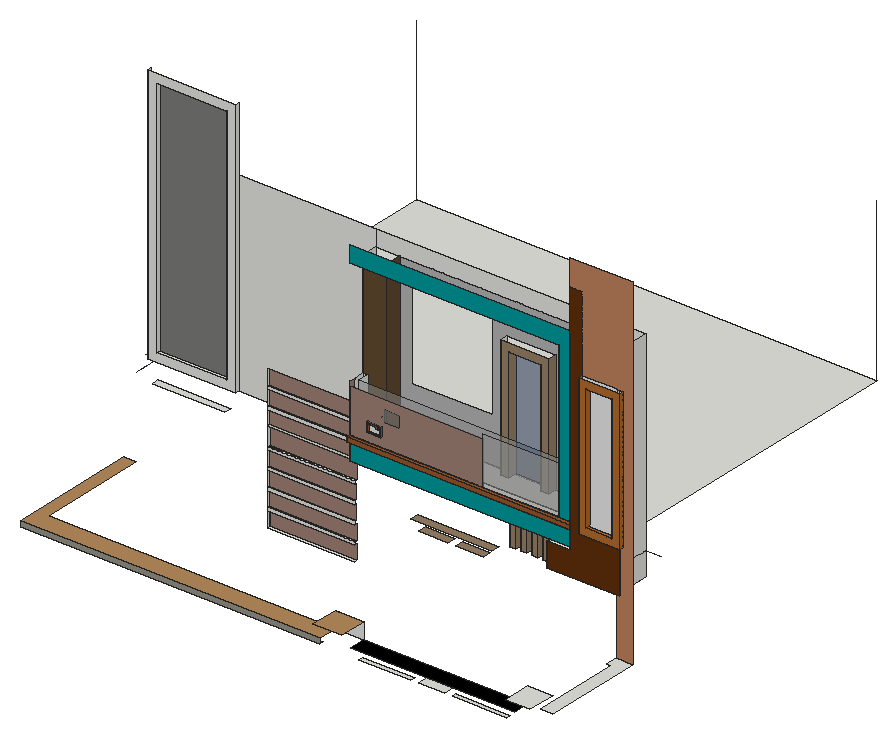
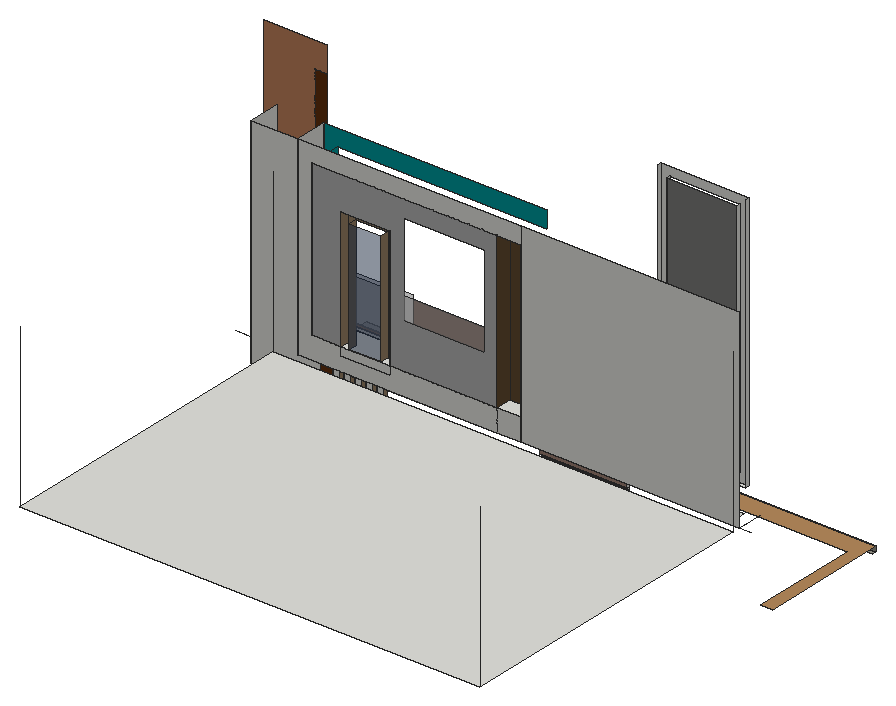
# SketchUp Ruby script. Lengths in inches.
U = 1.inch
M = Sketchup.active_model
def pt(a) = Geom::Point3d.new(a.map { |v| v * U })
def face(e, loops, mat)
  f = e.add_face(loops[0].map { |a| pt(a) })
  loops[1..].each { |l| e.add_face(l.map { |a| pt(a) }).erase! }
  f.material = f.back_material = mat if mat
  f
end
# faces: each face lists its corners as indices into pts; further lists are holes
def faces(e, pts, list, mat = nil) = list.each { |f| face(e, (f[0].is_a?(Array) ? f : [f]).map { |l| l.map { |i| pts[i] } }, mat) }
# xy, xz, yz: faces in a plane at the given z, y or x. An outline is a flat list of corners, or four numbers for a rectangle; further outlines are holes
def ring(l) = l.size == 4 ? [[l[0], l[1]], [l[2], l[1]], [l[2], l[3]], [l[0], l[3]]] : l.each_slice(2).to_a
def flat(e, list, mat, &to3) = list.each { |f| face(e, (f[0].is_a?(Array) ? f : [f]).map { |l| ring(l).map { |u, v| to3.(u, v) } }, mat) }
def xy(e, z, list, mat = nil) = flat(e, list, mat) { |x, y| [x, y, z] }
def xz(e, y, list, mat = nil) = flat(e, list, mat) { |x, z| [x, y, z] }
def yz(e, x, list, mat = nil) = flat(e, list, mat) { |y, z| [x, y, z] }
def lines(e, pts, list) = list.each { |a, b| e.add_line(pt(pts[a]), pt(pts[b])) }
# prism: a flat outline (further loops are holes) pulled along v
def prism(e, loops, v, mat = nil)
  f = face(e, loops, mat); d = Geom::Vector3d.new(v.map { |x| x * U })
  f.pushpull(f.normal.samedirection?(d) ? d.length : -d.length)
end
def box(e, o, s, mat = nil) = prism(e, [[o, [o[0] + s[0], o[1], o[2]], [o[0] + s[0], o[1] + s[1], o[2]], [o[0], o[1] + s[1], o[2]]]], [0, 0, s[2]], mat)
def at(x, y, z, deg = 0) = Geom::Transformation.translation(pt([x, y, z])) * Geom::Transformation.rotation(ORIGIN, Z_AXIS, deg.degrees)
def axes(o, x, y, z) = Geom::Transformation.new([*x, 0, *y, 0, *z, 0, *pt(o).to_a, 1])
def part(name) = M.definitions.add(name)
# library, detail: a bought-in or finely detailed component or shape, given as its bounding box
def library(name, o, s) = part(name).tap { |d| box(d.entities, o, s) }
def detail(e, o, s) = box(e.add_group.entities, o, s)
def put(e, d, t, mat = nil) = e.add_instance(d, t).tap { |i| i.material = mat if mat }
def group(e, t, mat = nil) = e.add_group.tap { |g| g.transformation = t; g.material = mat if mat }.entities
root = M.entities
M.materials.add("Niraj_Hair_Gray").color = [178, 178, 178]
M.materials.add("Niraj_Shoe_Sole").color = [96, 73, 48]
M.materials.add("Niraj_Shoe_Stitching").color = [181, 137, 92]
M.materials.add("Niraj_Skin").color = [158, 128, 115]
M.materials.add("[0035_Tan]").color = [150, 128, 100]
M.materials.add("[0043_SaddleBrown]").color = [96, 48, 13]
M.materials.add("[0083_DarkTurquoise]").color = [0, 153, 155]
M.materials.add("[0137_Black]").color = [0, 0, 0]
M.materials.add("[Basketweave]").color = [230, 230, 230]
M.materials.add("[Encaustic Tile Circular 01]").color = [123, 123, 122]
M.materials.add("[Formica Graystone]").color = [149, 146, 135]
M.materials.add("[Marble Carrara Gold Floor Tile]").color = [225, 223, 217]
M.materials.add("[Translucent Glass Blue]").color = [40, 60, 96]
M.materials["[Translucent Glass Blue]"].alpha = 0.5
M.materials.add("[Translucent Glass Gray]").color = [165, 165, 165]
M.materials["[Translucent Glass Gray]"].alpha = 0.5
M.materials.add("[Wood Bamboo]").color = [177, 105, 43]
M.materials.add("[Wood Cherry Original]").color = [152, 86, 42]
M.materials.add("[Wood Veneer 02]").color = [190, 128, 91]
xy(root,50.7,[[106.63,122.375,171.63,124.5]])
xy(root,54,[[249.65,28.875,288.24,31.875],[294.24,28.875,313.08,40.875],[319.08,28.875,359.58,31.875]])
xy(root,56.2,[[0,25.875,222.65,28.875]],"[Formica Graystone]")
xy(root,60,[[375,40.875,384,40.875,384,115,372,115,372,106,375,106]])
xy(root,60,[[0,25.875,222.65,25.875,222.65,40.875,9,40.875,9,122.375,0,122.375]],"Niraj_Shoe_Stitching")
xy(root,60,[[243.65,28.875,365.58,40.875]],"[0137_Black]")
xy(root,61.77,[[106.63,122.375,171.63,124.5]])
xy(root,64.2,[[106.63,122.375,171.63,123.875]])
xy(root,72,[[365.58,19.875,384,40.875]])
xy(root,72,[[222.65,19.875,243.65,40.875]],"Niraj_Shoe_Stitching")
xy(root,75.27,[[106.63,122.375,171.63,123.875]])
xy(root,77.7,[[106.63,122.375,171.63,123.5625]])
xy(root,78,[[208.6,136,229.96,142],[235.96,136,256.6,142]],"[0035_Tan]")
xy(root,84,[[202.6,136,262.6,142]],"[0035_Tan]")
xy(root,88.77,[[106.63,122.375,171.63,123.5625]])
xy(root,89.375,[[273.47,139,278.35,142],[281.66,139,286.54,142],[289.85,139,294.72,142],[298.04,139,302.91,142],[306.22,139,311.1,142]],"[0035_Tan]")
xy(root,91.2,[[106.63,122.375,171.63,123.5]])
xy(root,102.25,[[372,115,374.5,118]])
xy(root,102.25,[[320.38,115,372,142]],"[0043_SaddleBrown]")
xy(root,102.27,[[106.63,122.375,171.63,123.5]])
xy(root,104.7,[[106.63,122.375,171.63,123.9375],[106.63,123.9375,171.63,124.1875]])
xy(root,116.62,[[21.24,122.375,75.18,127.1875]])
xy(root,118.2,[[106.63,122.375,171.63,123.6875],[106.63,123.6875,171.63,124.1875]])
xy(root,120,[[320.38,115,337.38,118],[171.63,118,189.04,130],[320.38,118,337.38,142],[171.63,130,189.04,142],[273.47,139,278.35,142],
  [281.66,139,286.54,142],[289.85,139,294.72,142],[298.04,139,302.91,142],[306.22,139,311.1,142],[9,148,351,382.875]])
xy(root,120,[[189.04,118,189.04,142,273.47,142,273.47,139,278.35,139,278.35,142,281.66,142,281.66,139,286.54,139,286.54,142,289.85,142,289.85,139,294.72,139,294.72,142,298.04,142,298.04,139,302.91,139,302.91,142,306.22,142,306.22,139,311.1,139,311.1,142,320.38,142,320.38,118]],"[0083_DarkTurquoise]")
xy(root,129.27,[[106.63,122.375,171.63,123.6875]])
xy(root,131.7,[[106.63,122.375,171.63,123.9375]])
xy(root,133.71,[[171.63,115,337.38,118]],"[Wood Cherry Original]")
xy(root,134.02,[[20.16,119.375,85.33,122.375]])
xy(root,135.45,[[346.46,115,374.5,118],[374.5,115,376.65,118]])
xy(root,135.45,[[346.46,112,376.65,115]],"[Wood Bamboo]")
xy(root,136.875,[[171.63,118,171.63,130,175.07,130,175.07,122.125,326.57,122.125,326.57,118],[171.63,130,189.04,142],[269.26,136,275.26,142],[299.26,136,305.26,142]])
xy(root,136.875,[[175.07,122.125,326.57,122.125,326.57,142,305.26,142,305.26,136,299.26,136,299.26,142,275.26,142,275.26,136,269.26,136,269.26,142,189.04,142,189.04,130,175.07,130]],"[Marble Carrara Gold Floor Tile]")
xy(root,136.875,[[171.63,115,337.38,118]],"[Wood Cherry Original]")
xy(root,140.38,[[26.53,119.375,78.96,122.375]])
xy(root,140.875,[[351.89,112,371.22,118]],"[Wood Bamboo]")
xy(root,142.77,[[106.63,122.375,171.63,123.9375]])
xy(root,144.11,[[184.65,117,195.37,118]],"[Wood Cherry Original]")
xy(root,144.68,[[185.22,117,194.8,118]],"[Wood Cherry Original]")
xy(root,145.2,[[106.63,122.375,171.63,123.3125]])
xz(root,25.875,[[0,56.2,222.65,60]],"[Formica Graystone]")
xz(root,40.875,[[222.65,60,243.65,72]])
xz(root,112,[[[346.46,135.45,376.65,239.26],[351.89,140.875,371.22,233.83]]],"[Wood Bamboo]")
xz(root,115,[[372,135.45,374.5,239.26],[374.5,135.45,376.65,239.26]])
xz(root,115,[[320.38,102.25,374.5,102.25,374.5,135.45,346.46,135.45,346.46,295.34,337.38,295.34,337.38,120,320.38,120]],"[0043_SaddleBrown]")
xz(root,115,[[346.46,135.45,372,239.26]],"[Basketweave]")
xz(root,115,[[171.63,133.71,337.38,136.875]],"[Wood Cherry Original]")
xz(root,115,[[372,60,384,60,384,314.9,337.38,314.9,337.38,295.34,346.46,295.34,346.46,239.26,376.65,239.26,376.65,135.45,374.5,135.45,374.5,102.25,372,102.25]],"[Wood Veneer 02]")
xz(root,117,[[[184.65,144.11,195.37,150.73],[185.22,144.68,185.22,150.16,191.85,150.16,191.85,148.76,194.8,148.76,194.8,144.68],[192.49,149.21,194.8,150.16]]],"[Wood Cherry Original]")
xz(root,118,[[371.25,102.25,372,135.45],[372,102.25,374.5,135.45],[171.63,133.71,337.38,136.875],[346.46,135.45,371.25,239.26],[371.25,135.45,372,239.26],
  [372,135.45,374.5,239.26],[374.5,135.45,376.65,239.26],[351.89,140.875,371.22,233.83],[185.22,144.68,194.8,144.68,194.8,148.76,191.85,148.76,191.85,150.16,185.22,150.16]])
xz(root,118,[[[171.63,136.875,270.57,169.5625],[184.65,144.11,184.65,150.73,191.85,150.73,191.85,157.63,196.34,157.63,196.34,163.04,208.53,163.04,208.53,153.79,196.34,153.79,196.34,157.01,196.95,157.02,192.49,157.02,192.49,150.73,195.37,150.73,195.37,144.11]]],"Niraj_Skin")
xz(root,118,[[171.63,120,337.38,133.71],[326.57,136.875,337.38,136.875,337.38,264,171.63,264,171.63,251.8,326.57,251.8]],"[0083_DarkTurquoise]")
xz(root,118,[[270.57,136.875,326.57,172.875]],"[Translucent Glass Gray]")
xz(root,119.375,[[[20.16,134.02,85.33,326.3125],[26.53,140.38,78.96,319.95]]])
xz(root,122.125,[[175.07,136.875,326.57,172.875]],"[Translucent Glass Gray]")
xz(root,122.375,[[106.63,61.77,171.63,64.2],[106.63,75.27,171.63,77.7],[106.63,88.77,171.63,91.2],[106.63,102.27,171.63,104.7],[106.63,118.2,171.63,120],
  [106.63,129.27,171.63,131.7],[106.63,142.77,171.63,145.2]])
xz(root,122.375,[[26.53,140.38,78.96,319.95]],"[Encaustic Tile Circular 01]")
xz(root,123.3125,[[106.63,145.2,171.63,156.27]],"Niraj_Skin")
xz(root,123.5,[[106.63,91.2,171.63,102.27]],"Niraj_Skin")
xz(root,123.5625,[[106.63,77.7,171.63,88.77]],"Niraj_Skin")
xz(root,123.6875,[[106.63,118.2,171.63,129.27]],"Niraj_Skin")
xz(root,123.875,[[106.63,64.2,171.63,75.27]],"Niraj_Skin")
xz(root,123.9375,[[106.63,131.7,171.63,142.77]],"Niraj_Skin")
xz(root,124.1875,[[106.63,104.7,171.63,118.2]],"Niraj_Skin")
xz(root,124.5,[[106.63,50.7,171.63,61.77]],"Niraj_Skin")
xz(root,130,[[171.63,136.875,175.07,172.875]])
xz(root,130,[[175.07,136.875,189.04,136.875,189.04,251.8,171.63,251.8,171.63,172.875,175.07,172.875]],"Niraj_Shoe_Sole")
xz(root,136,[[269.26,136.875,275.26,136.875,275.26,220.875,299.26,220.875,299.26,136.875,305.26,136.875,305.26,226.875,269.26,226.875]],"[0035_Tan]")
xz(root,139,[[273.47,89.375,278.35,120],[281.66,89.375,286.54,120],[289.85,89.375,294.72,120],[298.04,89.375,302.91,120],[306.22,89.375,311.1,120]],"[0035_Tan]")
xz(root,142,[[273.47,89.375,278.35,120],[281.66,89.375,286.54,120],[289.85,89.375,294.72,120],[298.04,89.375,302.91,120],[306.22,89.375,311.1,120],
  [320.38,102.25,320.38,120,337.38,120,337.38,264,372,264,372,102.25],[9,120,171.63,264],[171.63,120,189.04,136.875],[189.04,120,337.38,120,337.38,264,171.63,264,171.63,251.8,326.57,251.8,326.57,136.875,305.26,136.875,305.26,130.875,269.26,130.875,269.26,136.875,189.04,136.875],[269.26,130.875,305.26,136.875]])
xz(root,142,[[[189.04,136.875,269.26,136.875,269.26,226.875,305.26,226.875,305.26,136.875,326.57,136.875,326.57,251.8,189.04,251.8],[198.26,170.25,258.45,239]]],"Niraj_Hair_Gray")
xz(root,142,[[275.26,136.875,299.26,220.875]],"[Translucent Glass Blue]")
yz(root,20.16,[[119.375,134.02,122.375,326.3125]])
yz(root,26.53,[[119.375,140.38,122.375,319.95]])
yz(root,78.96,[[119.375,140.38,122.375,319.95]])
yz(root,85.33,[[119.375,134.02,122.375,326.3125]])
yz(root,106.63,[[122.375,50.7,123.9375,61.77],[123.9375,50.7,124.5,61.77],[122.375,64.2,123.875,75.27],[123.875,64.2,124.5625,75.27],[122.375,77.7,123.5625,88.77],
  [123.5625,77.7,124.125,88.77],[122.375,91.2,123.5,102.27],[123.5,91.2,124.125,102.27],[122.375,104.7,124.1875,118.2],[122.375,118.2,123.6875,129.27],
  [122.375,131.7,123.9375,142.77],[122.375,145.2,123.3125,156.27]])
yz(root,171.63,[[122.375,118.2,123.6875,120],[123.6875,120,142,120,142,136.875,123.9375,136.875,123.9375,131.7,122.375,131.7,122.375,129.27,123.6875,129.27],[123.9375,136.875,123.9375,142.77,122.375,142.77,122.375,145.2,123.3125,145.2,123.3125,156.27,122.375,156.27,122.375,172.875,130,172.875,130,136.875],[130,136.875,142,251.8]])
yz(root,171.63,[[118,136.875,118,172.875,122.375,172.875,122.375,156.27,123.3125,156.27,123.3125,145.2,122.375,145.2,122.375,142.77,123.9375,142.77,123.9375,136.875]],"Niraj_Skin")
yz(root,171.63,[[118,120,118,136.875,123.9375,136.875,123.9375,131.7,122.375,131.7,122.375,129.27,123.6875,129.27,123.6875,120]],"[0083_DarkTurquoise]")
yz(root,171.63,[[115,133.71,118,136.875]],"[Wood Cherry Original]")
yz(root,175.07,[[122.125,136.875,130,172.875]])
yz(root,184.65,[[117,144.11,118,150.73]],"[Wood Cherry Original]")
yz(root,185.22,[[117,144.68,118,150.16]],"[Wood Cherry Original]")
yz(root,189.04,[[130,136.875,142,251.8]],"Niraj_Shoe_Sole")
yz(root,194.8,[[117,144.68,118,148.76]],"[Wood Cherry Original]")
yz(root,195.37,[[117,144.11,118,150.73]],"[Wood Cherry Original]")
yz(root,269.26,[[136,136.875,142,226.875]])
yz(root,273.47,[[139,89.375,142,120]],"[0035_Tan]")
yz(root,275.26,[[136,136.875,142,220.875]],"[0035_Tan]")
yz(root,278.35,[[139,89.375,142,120]],"[0035_Tan]")
yz(root,281.66,[[139,89.375,142,120]],"[0035_Tan]")
yz(root,286.54,[[139,89.375,142,120]],"[0035_Tan]")
yz(root,289.85,[[139,89.375,142,120]],"[0035_Tan]")
yz(root,294.72,[[139,89.375,142,120]],"[0035_Tan]")
yz(root,298.04,[[139,89.375,142,120]],"[0035_Tan]")
yz(root,299.26,[[136,136.875,142,220.875]],"[0035_Tan]")
yz(root,302.91,[[139,89.375,142,120]],"[0035_Tan]")
yz(root,305.26,[[136,136.875,142,226.875]],"[0035_Tan]")
yz(root,306.22,[[139,89.375,142,120]],"[0035_Tan]")
yz(root,311.1,[[139,89.375,142,120]],"[0035_Tan]")
yz(root,320.38,[[115,102.25,142,120]],"[0043_SaddleBrown]")
yz(root,326.57,[[118,136.875,122.125,172.875]])
yz(root,326.57,[[122.125,136.875,122.125,172.875,118,172.875,118,251.8,142,251.8,142,136.875]],"[0083_DarkTurquoise]")
yz(root,337.38,[[118,120,142,264],[115,133.71,118,136.875]])
yz(root,337.38,[[115,120,118,133.71],[115,136.875,118,264]],"[0043_SaddleBrown]")
yz(root,346.46,[[115,135.45,118,239.26]])
yz(root,346.46,[[112,135.45,115,239.26]],"[Wood Bamboo]")
yz(root,351.89,[[112,140.875,118,233.83]],"[Wood Bamboo]")
yz(root,371.22,[[112,140.875,118,233.83]],"[Wood Bamboo]")
yz(root,372,[[118,102.25,142,120],[118,120,142,264]])
yz(root,374.5,[[115,102.25,118,135.45]])
yz(root,376.65,[[115,135.45,118,239.26]])
yz(root,376.65,[[112,135.45,115,239.26]],"[Wood Bamboo]")
p = [[9,382.875,120],[9,382.875,240],[9,148,120],[9,148,240],[351,382.875,120],[351,382.875,240],
  [351,148,120],[351,148,240],[372,142,120],[384,142,120],[9,142,120],[0,142,120],
  [171.63,124.125,77.7],[106.63,124.125,77.7],[106.63,124.125,88.77],[171.63,124.125,88.77],[171.63,124.5625,64.2],[106.63,124.5625,64.2],
  [106.63,124.5625,75.27],[171.63,124.5625,75.27],[337.94,118,264],[337.94,118,102.25],[9,122.375,120]]
lines(root,p,[[0,1],[2,3],[4,5],[6,7],[8,9],[10,11],[12,13],[14,15],[16,17],[18,19],[20,21],[10,22]])
